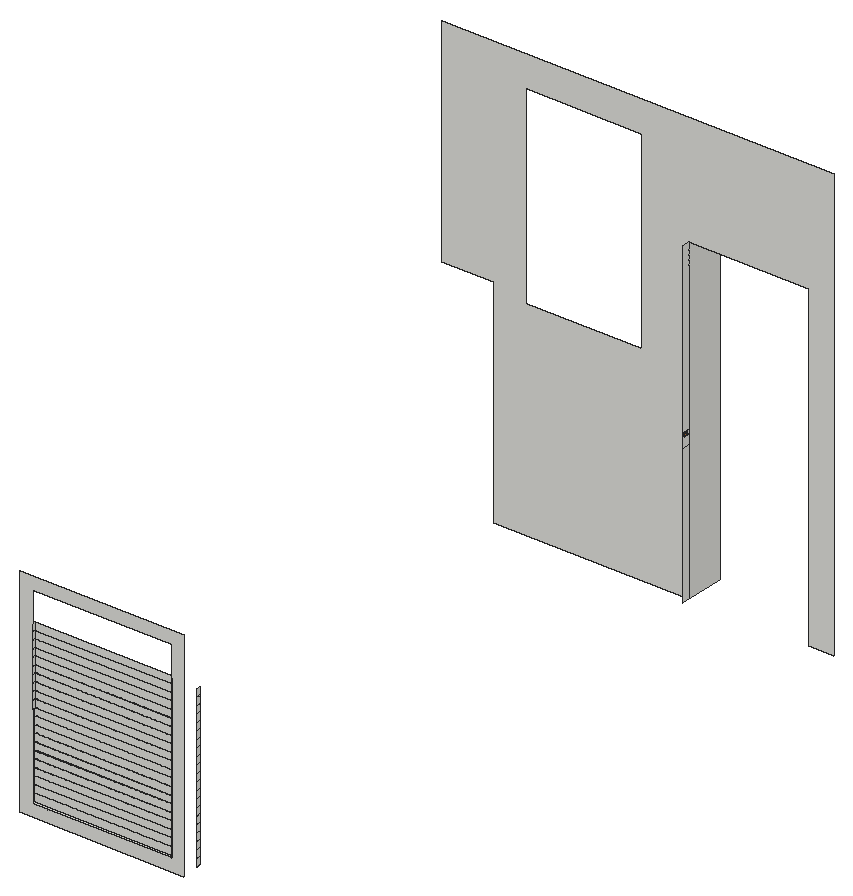
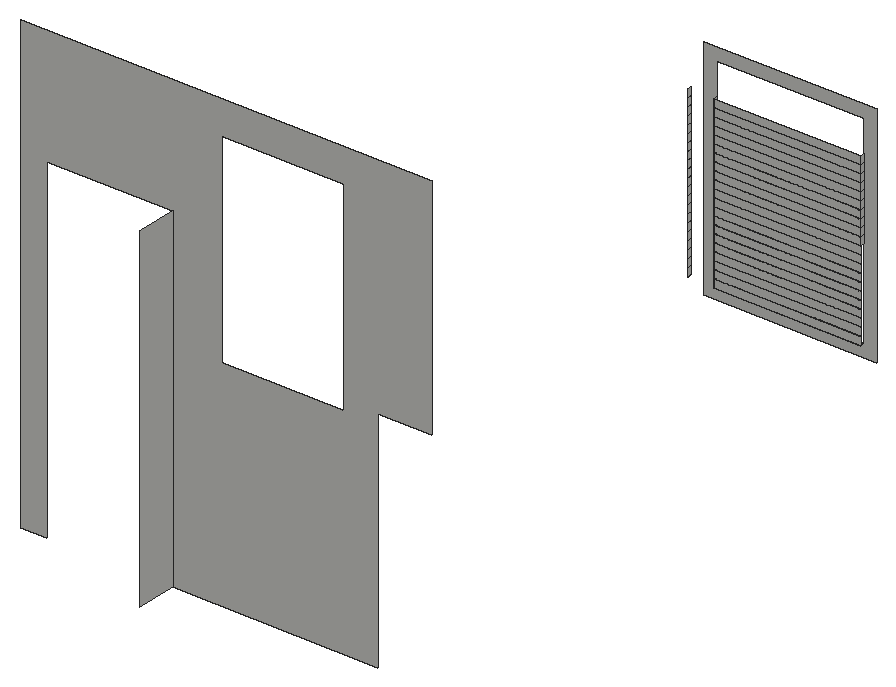
# SketchUp Ruby script. Lengths in inches.
U = 1.inch
M = Sketchup.active_model
def pt(a) = Geom::Point3d.new(a.map { |v| v * U })
def face(e, loops, mat)
  f = e.add_face(loops[0].map { |a| pt(a) })
  loops[1..].each { |l| e.add_face(l.map { |a| pt(a) }).erase! }
  f.material = f.back_material = mat if mat
  f
end
# faces: each face lists its corners as indices into pts; further lists are holes
def faces(e, pts, list, mat = nil) = list.each { |f| face(e, (f[0].is_a?(Array) ? f : [f]).map { |l| l.map { |i| pts[i] } }, mat) }
# xy, xz, yz: faces in a plane at the given z, y or x. An outline is a flat list of corners, or four numbers for a rectangle; further outlines are holes
def ring(l) = l.size == 4 ? [[l[0], l[1]], [l[2], l[1]], [l[2], l[3]], [l[0], l[3]]] : l.each_slice(2).to_a
def flat(e, list, mat, &to3) = list.each { |f| face(e, (f[0].is_a?(Array) ? f : [f]).map { |l| ring(l).map { |u, v| to3.(u, v) } }, mat) }
def xy(e, z, list, mat = nil) = flat(e, list, mat) { |x, y| [x, y, z] }
def xz(e, y, list, mat = nil) = flat(e, list, mat) { |x, z| [x, y, z] }
def yz(e, x, list, mat = nil) = flat(e, list, mat) { |y, z| [x, y, z] }
def lines(e, pts, list) = list.each { |a, b| e.add_line(pt(pts[a]), pt(pts[b])) }
# prism: a flat outline (further loops are holes) pulled along v
def prism(e, loops, v, mat = nil)
  f = face(e, loops, mat); d = Geom::Vector3d.new(v.map { |x| x * U })
  f.pushpull(f.normal.samedirection?(d) ? d.length : -d.length)
end
def box(e, o, s, mat = nil) = prism(e, [[o, [o[0] + s[0], o[1], o[2]], [o[0] + s[0], o[1] + s[1], o[2]], [o[0], o[1] + s[1], o[2]]]], [0, 0, s[2]], mat)
def at(x, y, z, deg = 0) = Geom::Transformation.translation(pt([x, y, z])) * Geom::Transformation.rotation(ORIGIN, Z_AXIS, deg.degrees)
def axes(o, x, y, z) = Geom::Transformation.new([*x, 0, *y, 0, *z, 0, *pt(o).to_a, 1])
def part(name) = M.definitions.add(name)
# library, detail: a bought-in or finely detailed component or shape, given as its bounding box
def library(name, o, s) = part(name).tap { |d| box(d.entities, o, s) }
def detail(e, o, s) = box(e.add_group.entities, o, s)
def put(e, d, t, mat = nil) = e.add_instance(d, t).tap { |i| i.material = mat if mat }
def group(e, t, mat = nil) = e.add_group.tap { |g| g.transformation = t; g.material = mat if mat }.entities
root = M.entities
M.materials.add("[Wood Bamboo]").color = [177, 105, 43]
xy(root,3.36,[[1101.82,64.97,1140.54,65.97]])
xz(root,64.97,[[[1098.46,0,1143.89,60],[1101.82,3.36,1140.54,56.64]]])
xz(root,65.97,[[1101.82,3.36,1140.54,5.49],[1101.82,5.49,1140.54,5.5],[1101.82,5.5,1140.54,7.62],[1101.82,7.62,1140.54,7.63],[1101.82,7.63,1140.54,9.75],
  [1101.82,9.75,1140.54,9.76],[1101.82,9.76,1140.54,11.88],[1101.82,11.88,1140.54,11.9],[1101.82,11.9,1140.54,14.01],[1101.82,14.01,1140.54,14.03],
  [1101.82,14.03,1140.54,16.14],[1101.82,16.14,1140.54,16.16],[1101.82,16.16,1140.54,18.27],[1101.82,18.27,1140.54,18.29],[1101.82,18.29,1140.54,20.4],
  [1101.82,20.4,1140.54,20.42],[1101.82,20.42,1140.54,22.53],[1101.82,22.53,1140.54,22.55],[1101.82,22.55,1140.54,24.66],[1101.82,24.66,1140.54,24.68],
  [1101.82,24.68,1140.54,26.8],[1101.82,26.8,1140.54,26.8125],[1101.82,26.8125,1140.54,28.93],[1101.82,28.93,1140.54,28.94],[1101.82,28.94,1140.54,31.06],
  [1101.82,31.06,1140.54,31.07],[1101.82,31.07,1140.54,33.1875],[1101.82,33.1875,1140.54,33.2],[1101.82,33.2,1140.54,35.32],[1101.82,35.32,1140.54,35.34],
  [1101.82,35.34,1140.54,37.45],[1101.82,37.45,1140.54,37.47],[1101.82,37.47,1140.54,39.58],[1101.82,39.58,1140.54,39.6],[1101.82,39.6,1140.54,41.71],
  [1101.82,41.71,1140.54,41.73],[1101.82,41.73,1140.54,43.84],[1101.82,43.84,1140.54,43.86],[1101.82,43.86,1140.54,45.97],[1101.82,45.97,1140.54,45.99],
  [1101.82,45.99,1140.54,48.1]])
xz(root,229.27,[[[1098.46,0,1152.79,0,1152.79,88.92,1186.04,88.92,1186.04,0,1192.93,0,1192.93,120,1084.25,120,1084.25,60,1098.46,60],[1107.5,57.5625,1139.63,111.3125]]])
yz(root,1101.82,[[64.97,26.8125,65.97,28.93],[64.97,28.93,65.97,28.94],[64.97,28.94,65.97,31.06],[64.97,31.06,65.97,31.07],[64.97,31.07,65.97,33.1875],
  [64.97,33.1875,65.97,33.2],[64.97,33.2,65.97,35.32],[64.97,35.32,65.97,35.34],[64.97,35.34,65.97,37.45],[64.97,37.45,65.97,37.47],
  [64.97,37.47,65.97,39.58],[64.97,39.58,65.97,39.6],[64.97,39.6,65.97,41.71],[64.97,41.71,65.97,41.73],[64.97,41.73,65.97,43.84],
  [64.97,43.84,65.97,43.86],[64.97,43.86,65.97,45.97],[64.97,45.97,65.97,45.99],[64.97,45.99,65.97,48.1]])
yz(root,1140.54,[[64.97,3.36,65.97,5.49],[64.97,5.49,65.97,5.5],[64.97,5.5,65.97,7.62],[64.97,7.62,65.97,7.63],[64.97,7.63,65.97,9.75],
  [64.97,9.75,65.97,9.76],[64.97,9.76,65.97,11.88],[64.97,11.88,65.97,11.9],[64.97,11.9,65.97,14.01],[64.97,14.01,65.97,14.03],
  [64.97,14.03,65.97,16.14],[64.97,16.14,65.97,16.16],[64.97,16.16,65.97,18.27],[64.97,18.27,65.97,18.29],[64.97,18.29,65.97,20.4],
  [64.97,20.4,65.97,20.42],[64.97,20.42,65.97,22.53],[64.97,22.53,65.97,22.55],[64.97,22.55,65.97,24.66],[64.97,24.66,65.97,24.68],
  [64.97,24.68,65.97,26.8],[64.97,26.8,65.97,26.8125],[64.97,26.8125,65.97,28.93],[64.97,28.93,65.97,28.94],[64.97,28.94,65.97,31.06],
  [64.97,31.06,65.97,31.07],[64.97,31.07,65.97,33.1875],[64.97,33.1875,65.97,33.2],[64.97,33.2,65.97,35.32],[64.97,35.32,65.97,35.34],
  [64.97,35.34,65.97,37.45],[64.97,37.45,65.97,37.47],[64.97,37.47,65.97,39.58],[64.97,39.58,65.97,39.6],[64.97,39.6,65.97,41.71],
  [64.97,41.71,65.97,41.73],[64.97,41.73,65.97,43.84],[64.97,43.84,65.97,43.86],[64.97,43.86,65.97,45.97],[64.97,45.97,65.97,45.99],
  [64.97,45.99,65.97,48.1]])
yz(root,1147.45,[[64.97,3.56,65.97,3.62],[64.97,3.62,65.97,5.73],[64.97,5.73,65.97,5.75],[64.97,5.75,65.97,7.85],[64.97,7.85,65.97,7.87],
  [64.97,7.87,65.97,9.96],[64.97,9.96,65.97,9.98],[64.97,9.98,65.97,12.07],[64.97,12.07,65.97,12.09],[64.97,12.09,65.97,14.18],
  [64.97,14.18,65.97,14.2],[64.97,14.2,65.97,16.29],[64.97,16.29,65.97,16.3125],[64.97,16.3125,65.97,18.41],[64.97,18.41,65.97,18.42],
  [64.97,18.42,65.97,20.52],[64.97,20.52,65.97,20.54],[64.97,20.54,65.97,22.63],[64.97,22.63,65.97,22.65],[64.97,22.65,65.97,24.74],
  [64.97,24.74,65.97,24.76],[64.97,24.76,65.97,26.85],[64.97,26.85,65.97,26.87],[64.97,26.87,65.97,28.97],[64.97,28.97,65.97,28.98],
  [64.97,28.98,65.97,31.08],[64.97,31.08,65.97,31.1],[64.97,31.1,65.97,33.19],[64.97,33.19,65.97,33.21],[64.97,33.21,65.97,35.3],
  [64.97,35.3,65.97,35.32],[64.97,35.32,65.97,37.41],[64.97,37.41,65.97,37.43],[64.97,37.43,65.97,39.53],[64.97,39.53,65.97,39.54],
  [64.97,39.54,65.97,41.64],[64.97,41.64,65.97,41.66],[64.97,41.66,65.97,43.75],[64.97,43.75,65.97,43.77],[64.97,43.77,65.97,45.86],
  [64.97,45.86,65.97,45.88],[64.97,45.88,65.97,47.97]])
yz(root,1152.79,[[227.27,0,229.27,38.29],[229.27,0,240.05,88.92],[227.27,38.29,229.27,88.92]])
p = [[1154,227.27,42.47],[1154.14,227.27,42.29],[1154.14,226.02,42.29],[1154,226.02,42.47],[1153.91,227.27,42.68],[1153.91,226.02,42.68],
  [1153.88,227.27,42.91],[1153.88,226.02,42.91],[1153.91,227.27,43.13],[1153.91,226.02,43.13],[1154,227.27,43.34],[1154,226.02,43.34],
  [1154.14,227.27,43.52],[1154.14,226.02,43.52]]
faces(root,p,[[0,1,2,3],[4,0,3,5],[6,4,5,7],[8,6,7,9],[10,8,9,11],[12,10,11,13]],"[Wood Bamboo]")
